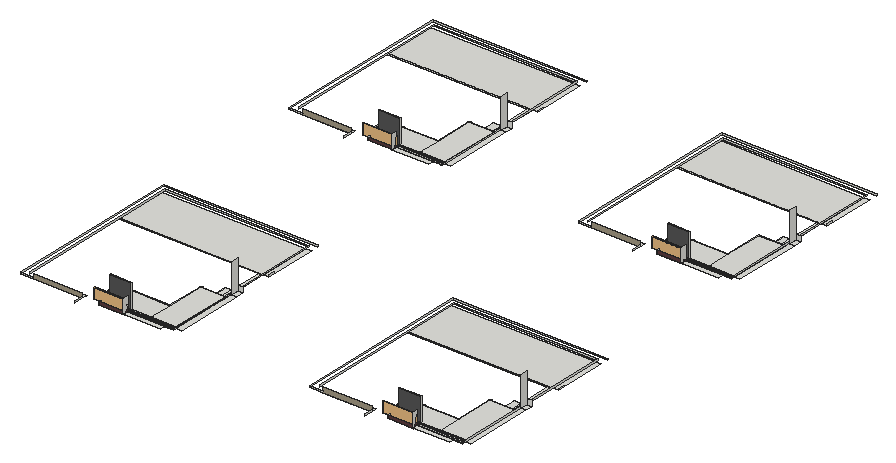
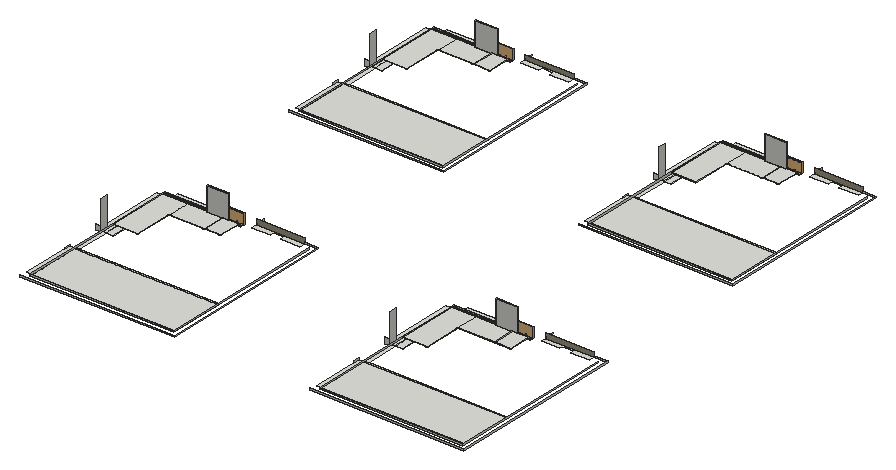
# SketchUp Ruby script. Lengths in inches.
U = 1.inch
M = Sketchup.active_model
def pt(a) = Geom::Point3d.new(a.map { |v| v * U })
def face(e, loops, mat)
  f = e.add_face(loops[0].map { |a| pt(a) })
  loops[1..].each { |l| e.add_face(l.map { |a| pt(a) }).erase! }
  f.material = f.back_material = mat if mat
  f
end
# faces: each face lists its corners as indices into pts; further lists are holes
def faces(e, pts, list, mat = nil) = list.each { |f| face(e, (f[0].is_a?(Array) ? f : [f]).map { |l| l.map { |i| pts[i] } }, mat) }
# xy, xz, yz: faces in a plane at the given z, y or x. An outline is a flat list of corners, or four numbers for a rectangle; further outlines are holes
def ring(l) = l.size == 4 ? [[l[0], l[1]], [l[2], l[1]], [l[2], l[3]], [l[0], l[3]]] : l.each_slice(2).to_a
def flat(e, list, mat, &to3) = list.each { |f| face(e, (f[0].is_a?(Array) ? f : [f]).map { |l| ring(l).map { |u, v| to3.(u, v) } }, mat) }
def xy(e, z, list, mat = nil) = flat(e, list, mat) { |x, y| [x, y, z] }
def xz(e, y, list, mat = nil) = flat(e, list, mat) { |x, z| [x, y, z] }
def yz(e, x, list, mat = nil) = flat(e, list, mat) { |y, z| [x, y, z] }
def lines(e, pts, list) = list.each { |a, b| e.add_line(pt(pts[a]), pt(pts[b])) }
# prism: a flat outline (further loops are holes) pulled along v
def prism(e, loops, v, mat = nil)
  f = face(e, loops, mat); d = Geom::Vector3d.new(v.map { |x| x * U })
  f.pushpull(f.normal.samedirection?(d) ? d.length : -d.length)
end
def box(e, o, s, mat = nil) = prism(e, [[o, [o[0] + s[0], o[1], o[2]], [o[0] + s[0], o[1] + s[1], o[2]], [o[0], o[1] + s[1], o[2]]]], [0, 0, s[2]], mat)
def at(x, y, z, deg = 0) = Geom::Transformation.translation(pt([x, y, z])) * Geom::Transformation.rotation(ORIGIN, Z_AXIS, deg.degrees)
def axes(o, x, y, z) = Geom::Transformation.new([*x, 0, *y, 0, *z, 0, *pt(o).to_a, 1])
def part(name) = M.definitions.add(name)
# library, detail: a bought-in or finely detailed component or shape, given as its bounding box
def library(name, o, s) = part(name).tap { |d| box(d.entities, o, s) }
def detail(e, o, s) = box(e.add_group.entities, o, s)
def put(e, d, t, mat = nil) = e.add_instance(d, t).tap { |i| i.material = mat if mat }
def group(e, t, mat = nil) = e.add_group.tap { |g| g.transformation = t; g.material = mat if mat }.entities
root = M.entities
M.materials.add("[Color M06]").color = [86, 86, 86]
M.materials.add("[Concrete Tile]").color = [165, 155, 133]
M.materials.add("[Granite Brown]").color = [89, 59, 61]
c1 = library("Glass Railing",[0,0,0],[139.5,4.76,42])
xy(root,370.6875,[[585.55,1810.0625,648.68,1834.0625],[1803.74,1810.0625,1866.87,1834.0625],[585.55,3224.75,648.68,3248.75],[1803.74,3224.75,1866.87,3248.75]])
xy(root,370.6875,[[648.68,1810.0625,695.43,1822.9375],[1866.87,1810.0625,1913.62,1822.9375],[648.68,3224.75,695.43,3237.625],[1866.87,3224.75,1913.62,3237.625]],"[Granite Brown]")
xy(root,377,[[648.68,1822.9375,648.68,1834.0625,557.88,1834.0625,557.88,1835.1875,890.875,1835.1875,890.875,1822.9375],[1866.87,1822.9375,1866.87,1834.0625,1776.07,1834.0625,1776.07,1835.1875,2109.0625,1835.1875,2109.0625,1822.9375],[648.68,3237.625,648.68,3248.75,557.88,3248.75,557.88,3249.875,890.875,3249.875,890.875,3237.625],[1866.87,3237.625,1866.87,3248.75,1776.07,3248.75,1776.07,3249.875,2109.0625,3249.875,2109.0625,3237.625]])
xy(root,378,[[320.25,1799.9375,320.25,1822.9375,400.51,1822.9375,400.51,1806.5625,445.4,1806.5625,445.4,1822.9375,523.04,1822.9375,523.04,1799.9375],[695.43,1799.9375,852.75,1822.9375],[1538.44,1799.9375,1538.44,1822.9375,1618.7,1822.9375,1618.7,1806.5625,1663.58,1806.5625,1663.58,1822.9375,1741.23,1822.9375,1741.23,1799.9375],[1913.62,1799.9375,2070.9375,1822.9375],[557.4,1835.1875,874.375,1839.6875],
  [874.375,1835.1875,890.875,1839.6875],[890.875,1835.1875,890.875,2148.83,894.3125,2148.83,894.3125,2124.51,913.875,2124.51,913.875,1835.1875],[1775.59,1835.1875,2092.5625,1839.6875],[2092.5625,1835.1875,2109.0625,1839.6875],[2109.0625,1835.1875,2109.0625,2148.83,2112.5,2148.83,2112.5,2124.51,2132.0625,2124.51,2132.0625,1835.1875],
  [846.5625,1839.6875,847.0625,2148.83],[847.0625,1839.6875,874.375,2148.83],[874.375,1839.6875,878.5625,2148.83],[878.5625,1839.6875,890.875,2148.83],[2064.75,1839.6875,2065.25,2148.83],
  [2065.25,1839.6875,2092.5625,2148.83],[2092.5625,1839.6875,2096.75,2148.83],[2096.75,1839.6875,2109.0625,2148.83],[894.3125,2124.51,913.875,2156.01],[2112.5,2124.51,2132.0625,2156.01],
  [874.375,2148.83,890.875,2290],[2092.5625,2148.83,2109.0625,2290],[285.875,2290,890.875,2295.875],[1504.0625,2290,2109.0625,2295.875],[285.875,2295.875,890.875,2518.89],
  [890.875,2295.875,913.875,2518.89],[1504.0625,2295.875,2109.0625,2518.89],[2109.0625,2295.875,2132.0625,2518.89],[320.25,3214.625,320.25,3237.625,400.51,3237.625,400.51,3221.25,445.4,3221.25,445.4,3237.625,523.04,3237.625,523.04,3214.625],[695.43,3214.625,852.75,3237.625],
  [1538.44,3214.625,1538.44,3237.625,1618.7,3237.625,1618.7,3221.25,1663.58,3221.25,1663.58,3237.625,1741.23,3237.625,1741.23,3214.625],[1913.62,3214.625,2070.9375,3237.625],[557.4,3249.875,874.375,3254.375],[874.375,3249.875,890.875,3254.375],[890.875,3249.875,890.875,3563.51,894.3125,3563.51,894.3125,3539.2,913.875,3539.2,913.875,3249.875],
  [1775.59,3249.875,2092.5625,3254.375],[2092.5625,3249.875,2109.0625,3254.375],[2109.0625,3249.875,2109.0625,3563.51,2112.5,3563.51,2112.5,3539.2,2132.0625,3539.2,2132.0625,3249.875],[846.5625,3254.375,847.0625,3563.51],[847.0625,3254.375,874.375,3563.51],
  [874.375,3254.375,878.5625,3563.51],[878.5625,3254.375,890.875,3563.51],[2064.75,3254.375,2065.25,3563.51],[2065.25,3254.375,2092.5625,3563.51],[2092.5625,3254.375,2096.75,3563.51],
  [2096.75,3254.375,2109.0625,3563.51],[894.3125,3539.2,913.875,3570.7],[2112.5,3539.2,2132.0625,3570.7],[874.375,3563.51,890.875,3704.6875],[2092.5625,3563.51,2109.0625,3704.6875],
  [285.875,3704.6875,890.875,3710.5625],[1504.0625,3704.6875,2109.0625,3710.5625],[285.875,3710.5625,890.875,3933.57],[890.875,3710.5625,913.875,3933.57],[1504.0625,3710.5625,2109.0625,3933.57],
  [2109.0625,3710.5625,2132.0625,3933.57]])
xy(root,379.5,[[648.68,1822.9375,648.68,1834.0625,632.49,1834.0625,632.49,1835.1875,890.875,1835.1875,890.875,1822.9375],[1866.87,1822.9375,1866.87,1834.0625,1850.67,1834.0625,1850.67,1835.1875,2109.0625,1835.1875,2109.0625,1822.9375],[648.68,3237.625,648.68,3248.75,632.49,3248.75,632.49,3249.875,890.875,3249.875,890.875,3237.625],[1866.87,3237.625,1866.87,3248.75,1850.67,3248.75,1850.67,3249.875,2109.0625,3249.875,2109.0625,3237.625]])
xy(root,383.25,[[564.5,1835.1875,632.49,1933.8125],[632.49,1835.1875,701.59,1839.6875],[701.59,1835.1875,701.59,1839.6875,632.49,1839.6875,632.49,1933.8125,784.3125,1933.8125,784.3125,1835.1875],[784.3125,1835.1875,890.875,2095.79],[1782.6875,1835.1875,1850.67,1933.8125],
  [1850.67,1835.1875,1919.77,1839.6875],[1919.77,1835.1875,1919.77,1839.6875,1850.67,1839.6875,1850.67,1933.8125,2002.5,1933.8125,2002.5,1835.1875],[2002.5,1835.1875,2109.0625,2095.79],[564.5,3249.875,632.49,3348.5],[632.49,3249.875,701.59,3254.375],
  [701.59,3249.875,701.59,3254.375,632.49,3254.375,632.49,3348.5,784.3125,3348.5,784.3125,3249.875],[784.3125,3249.875,890.875,3510.48],[1782.6875,3249.875,1850.67,3348.5],[1850.67,3249.875,1919.77,3254.375],[1919.77,3249.875,1919.77,3254.375,1850.67,3254.375,1850.67,3348.5,2002.5,3348.5,2002.5,3249.875],
  [2002.5,3249.875,2109.0625,3510.48]])
xz(root,1799.9375,[[262.875,378,319.53,384],[1481.0625,378,1537.72,384]])
xz(root,1799.9375,[[319.53,378,523.04,399.4375],[1537.72,378,1741.23,399.4375]],"[Concrete Tile]")
xz(root,1810.0625,[[585.55,370.6875,695.43,384],[1803.74,370.6875,1913.62,384]],"[Granite Brown]")
xz(root,1822.9375,[[695.43,377,852.75,378],[852.75,377,852.75,378,695.43,378,695.43,379.5,890.875,379.5,890.875,377],[1913.62,377,2070.9375,378],[2070.9375,377,2070.9375,378,1913.62,378,1913.62,379.5,2109.0625,379.5,2109.0625,377],[695.43,379.5,890.875,384],
  [1913.62,379.5,2109.0625,384]])
xz(root,1822.9375,[[648.68,370.6875,695.43,377],[1866.87,370.6875,1913.62,377],[648.68,377,695.43,379.5],[1866.87,377,1913.62,379.5]],"[Granite Brown]")
xz(root,1834.0625,[[585.55,370.6875,632.49,377],[632.49,370.6875,648.68,377],[1803.74,370.6875,1850.67,377],[1850.67,370.6875,1866.87,377],[557.88,377,585.55,384],
  [585.55,377,632.49,384],[632.49,377,648.68,379.5],[1776.07,377,1803.74,384],[1803.74,377,1850.67,384],[1850.67,377,1866.87,379.5]])
xz(root,1835.1875,[[557.4,377,874.375,378],[874.375,377,890.875,378],[1775.59,377,2092.5625,378],[2092.5625,377,2109.0625,378],[564.5,379.5,632.49,379.5,632.49,381.1875,611.65,381.1875,611.65,383.25,564.5,383.25],
  [632.49,379.5,632.49,381.1875,701.59,381.1875,701.59,383.25,890.875,383.25,890.875,379.5],[1782.6875,379.5,1850.67,379.5,1850.67,381.1875,1829.84,381.1875,1829.84,383.25,1782.6875,383.25],[1850.67,379.5,1850.67,381.1875,1919.77,381.1875,1919.77,383.25,2109.0625,383.25,2109.0625,379.5],[611.65,381.1875,632.49,383.25],[632.49,381.1875,701.59,383.25],
  [1829.84,381.1875,1850.67,383.25],[1850.67,381.1875,1919.77,383.25],[564.5,383.25,611.65,384],[611.65,383.25,632.49,384],[784.3125,383.25,890.875,384],
  [1782.6875,383.25,1829.84,384],[1829.84,383.25,1850.67,384],[2002.5,383.25,2109.0625,384]])
xz(root,1835.1875,[[632.49,383.25,701.59,383.25,701.59,481.8125,611.65,481.8125,611.65,384,632.49,384],[1850.67,383.25,1919.77,383.25,1919.77,481.8125,1829.84,481.8125,1829.84,384,1850.67,384]],"[Color M06]")
xz(root,1839.6875,[[632.49,383.25,632.49,384,611.65,384,611.65,481.8125,701.59,481.8125,701.59,383.25],[1850.67,383.25,1850.67,384,1829.84,384,1829.84,481.8125,1919.77,481.8125,1919.77,383.25]])
xz(root,1933.8125,[[564.5,383.25,632.49,384],[632.49,383.25,784.3125,384],[1782.6875,383.25,1850.67,384],[1850.67,383.25,2002.5,384]])
xz(root,2095.79,[[784.3125,383.25,890.875,384],[2002.5,383.25,2109.0625,384]])
xz(root,2156.01,[[894.3125,378,913.875,401.36],[2112.5,378,2132.0625,401.36]])
xz(root,2531.375,[[285.875,378,890.875,384],[1504.0625,378,2109.0625,384]])
xz(root,2554.375,[[262.875,378,913.875,384],[1481.0625,378,2132.0625,384]])
xz(root,3214.625,[[262.875,378,319.53,384],[1481.0625,378,1537.72,384]])
xz(root,3214.625,[[319.53,378,523.04,399.4375],[1537.72,378,1741.23,399.4375]],"[Concrete Tile]")
xz(root,3224.75,[[585.55,370.6875,695.43,384],[1803.74,370.6875,1913.62,384]],"[Granite Brown]")
xz(root,3237.625,[[695.43,377,852.75,378],[852.75,377,852.75,378,695.43,378,695.43,379.5,890.875,379.5,890.875,377],[1913.62,377,2070.9375,378],[2070.9375,377,2070.9375,378,1913.62,378,1913.62,379.5,2109.0625,379.5,2109.0625,377],[695.43,379.5,890.875,384],
  [1913.62,379.5,2109.0625,384]])
xz(root,3237.625,[[648.68,370.6875,695.43,377],[1866.87,370.6875,1913.62,377],[648.68,377,695.43,379.5],[1866.87,377,1913.62,379.5]],"[Granite Brown]")
xz(root,3248.75,[[585.55,370.6875,632.49,377],[632.49,370.6875,648.68,377],[1803.74,370.6875,1850.67,377],[1850.67,370.6875,1866.87,377],[557.88,377,585.55,384],
  [585.55,377,632.49,384],[632.49,377,648.68,379.5],[1776.07,377,1803.74,384],[1803.74,377,1850.67,384],[1850.67,377,1866.87,379.5]])
xz(root,3249.875,[[557.4,377,874.375,378],[874.375,377,890.875,378],[1775.59,377,2092.5625,378],[2092.5625,377,2109.0625,378],[564.5,379.5,632.49,379.5,632.49,381.1875,611.65,381.1875,611.65,383.25,564.5,383.25],
  [632.49,379.5,632.49,381.1875,701.59,381.1875,701.59,383.25,890.875,383.25,890.875,379.5],[1782.6875,379.5,1850.67,379.5,1850.67,381.1875,1829.84,381.1875,1829.84,383.25,1782.6875,383.25],[1850.67,379.5,1850.67,381.1875,1919.77,381.1875,1919.77,383.25,2109.0625,383.25,2109.0625,379.5],[611.65,381.1875,632.49,383.25],[632.49,381.1875,701.59,383.25],
  [1829.84,381.1875,1850.67,383.25],[1850.67,381.1875,1919.77,383.25],[564.5,383.25,611.65,384],[611.65,383.25,632.49,384],[784.3125,383.25,890.875,384],
  [1782.6875,383.25,1829.84,384],[1829.84,383.25,1850.67,384],[2002.5,383.25,2109.0625,384]])
xz(root,3249.875,[[632.49,383.25,701.59,383.25,701.59,481.8125,611.65,481.8125,611.65,384,632.49,384],[1850.67,383.25,1919.77,383.25,1919.77,481.8125,1829.84,481.8125,1829.84,384,1850.67,384]],"[Color M06]")
xz(root,3254.375,[[632.49,383.25,632.49,384,611.65,384,611.65,481.8125,701.59,481.8125,701.59,383.25],[1850.67,383.25,1850.67,384,1829.84,384,1829.84,481.8125,1919.77,481.8125,1919.77,383.25]])
xz(root,3348.5,[[564.5,383.25,632.49,384],[632.49,383.25,784.3125,384],[1782.6875,383.25,1850.67,384],[1850.67,383.25,2002.5,384]])
xz(root,3510.48,[[784.3125,383.25,890.875,384],[2002.5,383.25,2109.0625,384]])
xz(root,3570.7,[[894.3125,378,913.875,401.36],[2112.5,378,2132.0625,401.36]])
xz(root,3946.0625,[[285.875,378,890.875,384],[1504.0625,378,2109.0625,384]])
xz(root,3969.0625,[[262.875,378,913.875,384],[1481.0625,378,2132.0625,384]])
yz(root,262.875,[[1799.9375,378,2554.375,384],[3214.625,378,3969.0625,384]])
yz(root,285.875,[[1822.9375,378,2531.375,384],[3237.625,378,3946.0625,384]])
yz(root,523.04,[[1763.25,378,1799.9375,384],[3177.9375,378,3214.625,384]])
yz(root,564.5,[[1835.1875,383.25,1836.0625,384],[1836.0625,383.25,1837.8125,384],[1837.8125,383.25,1933.8125,384],[3249.875,383.25,3250.75,384],[3250.75,383.25,3252.5,384],
  [3252.5,383.25,3348.5,384]])
yz(root,585.55,[[1810.0625,370.6875,1834.0625,384],[3224.75,370.6875,3248.75,384]])
yz(root,632.49,[[1834.0625,379.5,1835.1875,384],[3248.75,379.5,3249.875,384],[1835.1875,383.25,1839.6875,384],[1839.6875,383.25,1933.8125,384],[3249.875,383.25,3254.375,384],
  [3254.375,383.25,3348.5,384]])
yz(root,648.68,[[1822.9375,370.6875,1834.0625,377],[3237.625,370.6875,3248.75,377],[1822.9375,377,1834.0625,379.5],[3237.625,377,3248.75,379.5]])
yz(root,695.43,[[1799.9375,378,1799.9375,435.5,1822.9375,435.5,1822.9375,384,1810.0625,384,1810.0625,378],[3214.625,378,3214.625,435.5,3237.625,435.5,3237.625,384,3224.75,384,3224.75,378]])
yz(root,695.43,[[1810.0625,370.6875,1822.9375,378],[3224.75,370.6875,3237.625,378],[1810.0625,378,1822.9375,384],[3224.75,378,3237.625,384]],"[Granite Brown]")
yz(root,701.59,[[1835.1875,383.25,1839.6875,481.8125],[3249.875,383.25,3254.375,481.8125]])
yz(root,784.3125,[[1933.8125,383.25,2095.79,384],[3348.5,383.25,3510.48,384]])
yz(root,890.875,[[1822.9375,377,1822.9375,379.5,1835.1875,379.5,1835.1875,383.25,2095.79,383.25,2095.79,384,2531.375,384,2531.375,378,1835.1875,378,1835.1875,377],[3237.625,377,3237.625,379.5,3249.875,379.5,3249.875,383.25,3510.48,383.25,3510.48,384,3946.0625,384,3946.0625,378,3249.875,378,3249.875,377],[1822.9375,379.5,1835.1875,384],[3237.625,379.5,3249.875,384],[1835.1875,383.25,2095.79,384],
  [3249.875,383.25,3510.48,384]])
yz(root,894.3125,[[2124.51,378,2156.01,504],[3539.2,378,3570.7,504]])
yz(root,913.875,[[2295.875,378,2321.98,384],[3710.5625,378,3736.67,384]])
yz(root,1481.0625,[[1799.9375,378,2554.375,384],[3214.625,378,3969.0625,384]])
yz(root,1504.0625,[[1822.9375,378,2531.375,384],[3237.625,378,3946.0625,384]])
yz(root,1741.23,[[1763.25,378,1799.9375,384],[3177.9375,378,3214.625,384]])
yz(root,1782.6875,[[1835.1875,383.25,1836.0625,384],[1836.0625,383.25,1837.8125,384],[1837.8125,383.25,1933.8125,384],[3249.875,383.25,3250.75,384],[3250.75,383.25,3252.5,384],
  [3252.5,383.25,3348.5,384]])
yz(root,1803.74,[[1810.0625,370.6875,1834.0625,384],[3224.75,370.6875,3248.75,384]])
yz(root,1850.67,[[1834.0625,379.5,1835.1875,384],[3248.75,379.5,3249.875,384],[1835.1875,383.25,1839.6875,384],[1839.6875,383.25,1933.8125,384],[3249.875,383.25,3254.375,384],
  [3254.375,383.25,3348.5,384]])
yz(root,1866.87,[[1822.9375,370.6875,1834.0625,377],[3237.625,370.6875,3248.75,377],[1822.9375,377,1834.0625,379.5],[3237.625,377,3248.75,379.5]])
yz(root,1913.62,[[1799.9375,378,1799.9375,435.5,1822.9375,435.5,1822.9375,384,1810.0625,384,1810.0625,378],[3214.625,378,3214.625,435.5,3237.625,435.5,3237.625,384,3224.75,384,3224.75,378]])
yz(root,1913.62,[[1810.0625,370.6875,1822.9375,378],[3224.75,370.6875,3237.625,378],[1810.0625,378,1822.9375,384],[3224.75,378,3237.625,384]],"[Granite Brown]")
yz(root,1919.77,[[1835.1875,383.25,1839.6875,481.8125],[3249.875,383.25,3254.375,481.8125]])
yz(root,2002.5,[[1933.8125,383.25,2095.79,384],[3348.5,383.25,3510.48,384]])
yz(root,2109.0625,[[1822.9375,377,1822.9375,379.5,1835.1875,379.5,1835.1875,383.25,2095.79,383.25,2095.79,384,2531.375,384,2531.375,378,1835.1875,378,1835.1875,377],[3237.625,377,3237.625,379.5,3249.875,379.5,3249.875,383.25,3510.48,383.25,3510.48,384,3946.0625,384,3946.0625,378,3249.875,378,3249.875,377],[1822.9375,379.5,1835.1875,384],[3237.625,379.5,3249.875,384],[1835.1875,383.25,2095.79,384],
  [3249.875,383.25,3510.48,384]])
yz(root,2112.5,[[2124.51,378,2156.01,504],[3539.2,378,3570.7,504]])
yz(root,2132.0625,[[2295.875,378,2321.98,384],[3710.5625,378,3736.67,384]])
p = [[1537.72,1778.3125,378],[1538.44,1778.3125,378],[1741.23,1778.3125,378],[1741.23,1778.3125,384],[319.53,1778.3125,378],[320.25,1778.3125,378],
  [523.04,1778.3125,378],[523.04,1778.3125,384],[1537.72,3193,378],[1538.44,3193,378],[1741.23,3193,378],[1741.23,3193,384],
  [319.53,3193,378],[320.25,3193,378],[523.04,3193,378],[523.04,3193,384]]
lines(root,p,[[0,1],[2,3],[4,5],[6,7],[8,9],[10,11],[12,13],[14,15]])
put(root,c1,at(1774.12,1820.19,377.3125),"[Color M06]")
put(root,c1,at(555.93,1820.19,377.3125),"[Color M06]")
put(root,c1,at(1774.12,3234.88,377.3125),"[Color M06]")
put(root,c1,at(555.93,3234.88,377.3125),"[Color M06]")
